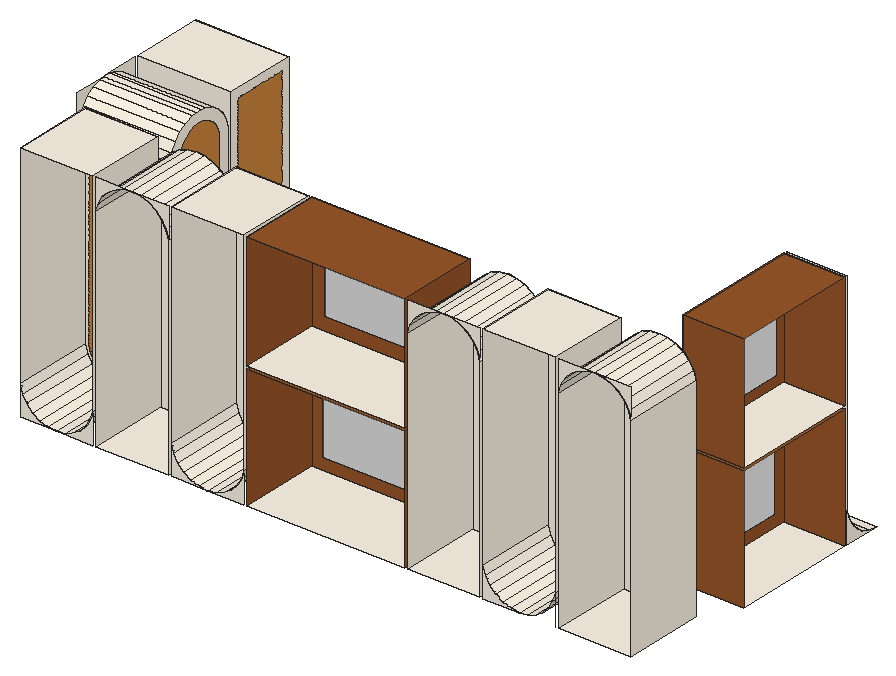
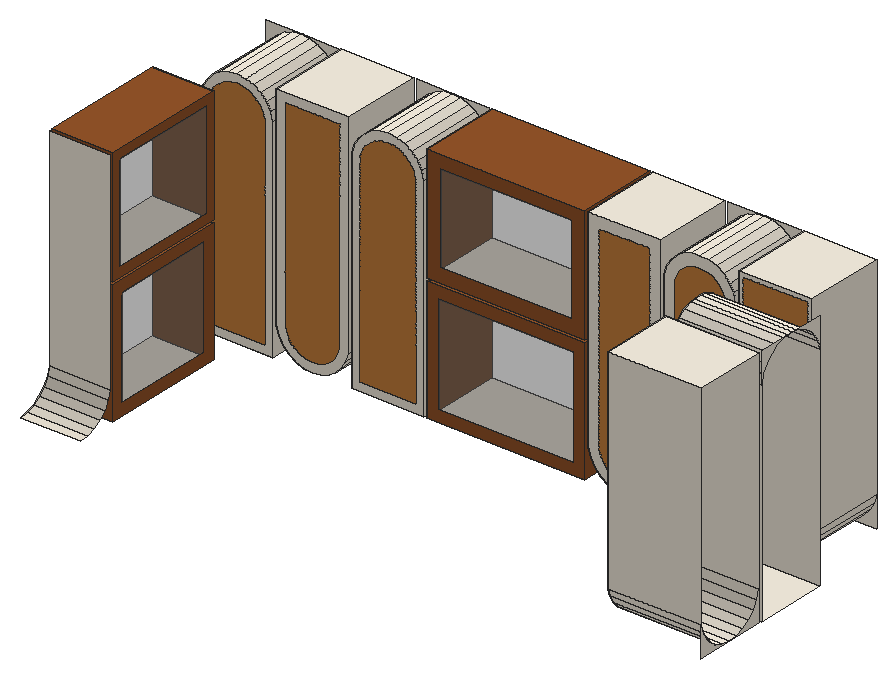
# SketchUp Ruby script. Lengths in inches.
U = 1.inch
M = Sketchup.active_model
def pt(a) = Geom::Point3d.new(a.map { |v| v * U })
def face(e, loops, mat)
  f = e.add_face(loops[0].map { |a| pt(a) })
  loops[1..].each { |l| e.add_face(l.map { |a| pt(a) }).erase! }
  f.material = f.back_material = mat if mat
  f
end
# faces: each face lists its corners as indices into pts; further lists are holes
def faces(e, pts, list, mat = nil) = list.each { |f| face(e, (f[0].is_a?(Array) ? f : [f]).map { |l| l.map { |i| pts[i] } }, mat) }
# xy, xz, yz: faces in a plane at the given z, y or x. An outline is a flat list of corners, or four numbers for a rectangle; further outlines are holes
def ring(l) = l.size == 4 ? [[l[0], l[1]], [l[2], l[1]], [l[2], l[3]], [l[0], l[3]]] : l.each_slice(2).to_a
def flat(e, list, mat, &to3) = list.each { |f| face(e, (f[0].is_a?(Array) ? f : [f]).map { |l| ring(l).map { |u, v| to3.(u, v) } }, mat) }
def xy(e, z, list, mat = nil) = flat(e, list, mat) { |x, y| [x, y, z] }
def xz(e, y, list, mat = nil) = flat(e, list, mat) { |x, z| [x, y, z] }
def yz(e, x, list, mat = nil) = flat(e, list, mat) { |y, z| [x, y, z] }
def lines(e, pts, list) = list.each { |a, b| e.add_line(pt(pts[a]), pt(pts[b])) }
# prism: a flat outline (further loops are holes) pulled along v
def prism(e, loops, v, mat = nil)
  f = face(e, loops, mat); d = Geom::Vector3d.new(v.map { |x| x * U })
  f.pushpull(f.normal.samedirection?(d) ? d.length : -d.length)
end
def box(e, o, s, mat = nil) = prism(e, [[o, [o[0] + s[0], o[1], o[2]], [o[0] + s[0], o[1] + s[1], o[2]], [o[0], o[1] + s[1], o[2]]]], [0, 0, s[2]], mat)
def at(x, y, z, deg = 0) = Geom::Transformation.translation(pt([x, y, z])) * Geom::Transformation.rotation(ORIGIN, Z_AXIS, deg.degrees)
def axes(o, x, y, z) = Geom::Transformation.new([*x, 0, *y, 0, *z, 0, *pt(o).to_a, 1])
def part(name) = M.definitions.add(name)
# library, detail: a bought-in or finely detailed component or shape, given as its bounding box
def library(name, o, s) = part(name).tap { |d| box(d.entities, o, s) }
def detail(e, o, s) = box(e.add_group.entities, o, s)
def put(e, d, t, mat = nil) = e.add_instance(d, t).tap { |i| i.material = mat if mat }
def group(e, t, mat = nil) = e.add_group.tap { |g| g.transformation = t; g.material = mat if mat }.entities
root = M.entities
M.materials.add("[0030_OldLace]").color = [253, 245, 230]
M.materials.add("[0040_Peru]").color = [205, 133, 63]
M.materials.add("[Translucent Glass Gray]").color = [128, 128, 128]
M.materials["[Translucent Glass Gray]"].alpha = 0.5
M.materials.add("[Wood Cherry Original]").color = [152, 86, 42]
xy(root,67.4375,[[9,29.46,24.375,41.46]],"[0030_OldLace]")
xy(root,67.6875,[[24.875,13.46,36.875,26.84],[49.875,13.46,76,26.84],[76.5,13.46,88.5,26.84],[101.5,13.46,113.5,26.84]],"[0030_OldLace]")
xy(root,67.8125,[[106.9375,32.34,117,53.28]],"[0030_OldLace]")
xy(root,87.9375,[[49.875,13.46,76,26.84]],"[Wood Cherry Original]")
xy(root,88.125,[[106.9375,32.34,117,53.28]],"[Wood Cherry Original]")
xy(root,88.4375,[[49.875,13.46,76,26.84]],"[0030_OldLace]")
xy(root,88.625,[[106.9375,32.34,117,53.28]],"[0030_OldLace]")
xy(root,107.5625,[[9,34.93,24.375,36],[9,41.96,24.375,53.96]],"[0030_OldLace]")
xy(root,107.625,[[12.375,13.46,24.375,26.84],[37.375,13.46,49.375,26.84]],"[0030_OldLace]")
xy(root,107.625,[[49.875,13.46,76,26.84]],"[Wood Cherry Original]")
xy(root,107.6875,[[89,13.46,101,26.84]],"[0030_OldLace]")
xy(root,107.6875,[[106.9375,32.34,117,53.28]],"[Wood Cherry Original]")
xz(root,13.46,[[12.375,67.6875,12.375,72.6875,12.79,71.34,13.5,70.12,14.47,69.1,15.65,68.33,16.97,67.85,18.375,67.6875],[18.375,67.6875,19.78,67.85,21.1,68.33,22.28,69.1,23.25,70.12,23.96,71.34,24.375,72.6875,24.375,67.6875],[37.375,67.6875,37.375,72.6875,37.79,71.34,38.5,70.12,39.47,69.1,40.65,68.33,41.97,67.85,43.375,67.6875],[43.375,67.6875,44.78,67.85,46.1,68.33,47.28,69.1,48.25,70.12,48.96,71.34,49.375,72.6875,49.375,67.6875],[89,67.6875,89,72.6875,89.41,71.34,90.125,70.12,91.09,69.1,92.27,68.33,93.6,67.85,95,67.6875],
  [24.875,102.625,24.875,107.625,30.875,107.625,29.47,107.46,28.15,106.98,26.97,106.21,26,105.19,25.29,103.97],[36.875,102.625,36.46,103.97,35.75,105.19,34.78,106.21,33.6,106.98,32.28,107.46,30.875,107.625,36.875,107.625],[76.5,102.625,76.5,107.625,82.5,107.625,81.1,107.46,79.77,106.98,78.59,106.21,77.625,105.19,76.91,103.97],[88.5,102.625,88.09,103.97,87.375,105.19,86.41,106.21,85.23,106.98,83.9,107.46,82.5,107.625,88.5,107.625],[101.5,102.625,101.5,107.625,107.5,107.625,106.1,107.46,104.77,106.98,103.59,106.21,102.625,105.19,101.91,103.97],
  [113.5,102.625,113.09,103.97,112.375,105.19,111.41,106.21,110.23,106.98,108.9,107.46,107.5,107.625,113.5,107.625]],"[0030_OldLace]")
xz(root,26.84,[[[18.375,67.6875,16.97,67.85,15.65,68.33,14.47,69.1,13.5,70.12,12.79,71.34,12.375,72.6875,12.375,107.625,24.375,107.625,24.375,72.6875,23.96,71.34,23.25,70.12,22.28,69.1,21.1,68.33,19.78,67.85],[18.375,68.33,19.625,68.48,20.8125,68.91,21.87,69.6,22.73,70.51,23.37,71.6,23.73,72.78,23.73,106.98,13.02,106.98,13.02,72.78,13.38,71.6,14.02,70.51,14.88,69.6,15.9375,68.91,17.125,68.48]],[[24.875,67.6875,24.875,102.625,25.29,103.97,26,105.19,26.97,106.21,28.15,106.98,29.47,107.46,30.875,107.625,32.28,107.46,33.6,106.98,34.78,106.21,35.75,105.19,36.46,103.97,36.875,102.625,36.875,67.6875],[26.64,69.46,35.11,69.46,35.11,102.36,34.83,103.26,34.33,104.12,33.64,104.84,32.8,105.39,31.87,105.73,30.875,105.84,29.88,105.73,28.95,105.39,28.11,104.84,27.42,104.12,26.92,103.26,26.64,102.36]],[[43.375,67.6875,41.97,67.85,40.65,68.33,39.47,69.1,38.5,70.12,37.79,71.34,37.375,72.6875,37.375,107.625,49.375,107.625,49.375,72.6875,48.96,71.34,48.25,70.12,47.28,69.1,46.1,68.33,44.78,67.85],[43.375,69.56,44.35,69.67,45.26,70,46.08,70.54,46.76,71.25,47.25,72.09,47.52,72.97,47.52,105.77,39.23,105.77,39.23,72.97,39.5,72.09,39.99,71.25,40.67,70.54,41.49,70,42.4,69.67]],[[76.5,67.6875,76.5,102.625,76.91,103.97,77.625,105.19,78.59,106.21,79.77,106.98,81.1,107.46,82.5,107.625,83.9,107.46,85.23,106.98,86.41,106.21,87.375,105.19,88.09,103.97,88.5,102.625,88.5,67.6875],[77.875,69.0625,87.125,69.0625,87.125,102.42,86.82,103.42,86.27,104.36,85.52,105.15,84.61,105.74,83.58,106.12,82.5,106.24,81.42,106.12,80.39,105.74,79.48,105.15,78.73,104.36,78.18,103.42,77.875,102.42]],[[95,67.6875,93.6,67.85,92.27,68.33,91.09,69.1,90.125,70.12,89.41,71.34,89,72.6875,89,107.6875,101,107.6875,101,72.6875,100.59,71.34,99.875,70.12,98.91,69.1,97.73,68.33,96.4,67.85],[95,69.14,96.07,69.26,97.08,69.625,97.98,70.21,98.72,70.99,99.26,71.92,99.5625,72.9,99.5625,106.25,90.4375,106.25,90.4375,72.9,90.74,71.92,91.28,70.99,92.02,70.21,92.92,69.625,93.93,69.26]],
  [[101.5,67.6875,101.5,102.625,101.91,103.97,102.625,105.19,103.59,106.21,104.77,106.98,106.1,107.46,107.5,107.625,108.9,107.46,110.23,106.98,111.41,106.21,112.375,105.19,113.09,103.97,113.5,102.625,113.5,67.6875],[102.875,69.0625,112.125,69.0625,112.125,102.42,111.82,103.42,111.27,104.36,110.52,105.15,109.61,105.75,108.58,106.12,107.5,106.24,106.42,106.12,105.39,105.75,104.48,105.15,103.73,104.36,103.18,103.42,102.875,102.42]]],"[0030_OldLace]")
xz(root,26.84,[[18.375,68.33,17.125,68.48,15.9375,68.91,14.88,69.6,14.02,70.51,13.38,71.6,13.02,72.78,13.02,106.98,23.73,106.98,23.73,72.78,23.37,71.6,22.73,70.51,21.87,69.6,20.8125,68.91,19.625,68.48],[77.875,69.0625,77.875,102.42,78.18,103.42,78.73,104.36,79.48,105.15,80.39,105.74,81.42,106.12,82.5,106.24,83.58,106.12,84.61,105.74,85.52,105.15,86.27,104.36,86.82,103.42,87.125,102.42,87.125,69.0625],[102.875,69.0625,102.875,102.42,103.18,103.42,103.73,104.36,104.48,105.15,105.39,105.75,106.42,106.12,107.5,106.24,108.58,106.12,109.61,105.75,110.52,105.15,111.27,104.36,111.82,103.42,112.125,102.42,112.125,69.0625],[95,69.14,93.93,69.26,92.92,69.625,92.02,70.21,91.28,70.99,90.74,71.92,90.4375,72.9,90.4375,106.25,99.5625,106.25,99.5625,72.9,99.26,71.92,98.72,70.99,97.98,70.21,97.08,69.625,96.07,69.26],[26.64,69.46,26.64,102.36,26.92,103.26,27.42,104.12,28.11,104.84,28.95,105.39,29.88,105.73,30.875,105.84,31.87,105.73,32.8,105.39,33.64,104.84,34.33,104.12,34.83,103.26,35.11,102.36,35.11,69.46],
  [43.375,69.56,42.4,69.67,41.49,70,40.67,70.54,39.99,71.25,39.5,72.09,39.23,72.97,39.23,105.77,47.52,105.77,47.52,72.97,47.25,72.09,46.76,71.25,46.08,70.54,45.26,70,44.35,69.67]],"[0040_Peru]")
xz(root,26.84,[[51.76,69.57,74.11,86.05],[52.125,90.6875,73.75,105.375]],"[Translucent Glass Gray]")
xz(root,26.84,[[[49.875,67.6875,76,87.9375],[51.76,69.57,74.11,86.05]],[[49.875,88.4375,76,107.625],[52.125,90.6875,73.75,105.375]]],"[Wood Cherry Original]")
xz(root,29.46,[[9,67.4375,24.375,102.5625]],"[0030_OldLace]")
xz(root,32.34,[[106.9375,67.8125,117,88.125],[106.9375,88.625,117,107.6875]],"[Wood Cherry Original]")
xz(root,41.46,[[9,67.4375,24.375,102.5625]],"[0030_OldLace]")
xz(root,41.96,[[9,72.4375,24.375,107.5625]],"[0030_OldLace]")
xz(root,53.28,[[106.9375,67.8125,117,88.125],[106.9375,88.625,117,107.6875]],"[Wood Cherry Original]")
xz(root,53.78,[[106.9375,72.8125,117,107.6875]],"[0030_OldLace]")
xz(root,53.96,[[9,72.4375,24.375,107.5625]],"[0030_OldLace]")
yz(root,9,[[41.96,67.4375,47.96,67.4375,46.56,67.6,45.24,68.08,44.06,68.85,43.09,69.87,42.38,71.09,41.96,72.4375],[47.96,67.4375,53.96,67.4375,53.96,72.4375,53.55,71.09,52.84,69.87,51.87,68.85,50.69,68.08,49.36,67.6],[29.46,102.5625,29.87,103.92,30.57,105.16,31.54,106.19,32.72,106.97,34.06,107.46,34.93,107.5625,29.46,107.5625],[41.46,102.5625,41.46,107.5625,36,107.5625,36.875,107.46,38.21,106.97,39.39,106.19,40.36,105.16,41.06,103.92],[34.93,107.5625,36,107.5625,35.46,107.625]],"[0030_OldLace]")
yz(root,12.375,[[13.46,72.6875,26.84,107.625]],"[0030_OldLace]")
yz(root,24.375,[[[29.46,67.4375,41.46,67.4375,41.46,102.5625,41.06,103.92,40.36,105.16,39.39,106.19,38.21,106.97,36.875,107.46,36,107.5625,34.93,107.5625,34.06,107.46,32.72,106.97,31.54,106.19,30.57,105.16,29.87,103.92,29.46,102.5625],[31.14,69.11,31.14,102.32,31.41,103.26,31.92,104.16,32.625,104.9,33.48,105.47,34.45,105.82,35.03,105.89,35.9,105.89,36.48,105.82,37.45,105.47,38.31,104.9,39.01,104.16,39.52,103.26,39.79,102.32,39.79,69.11]],[[47.96,67.4375,49.36,67.6,50.69,68.08,51.87,68.85,52.84,69.87,53.55,71.09,53.96,72.4375,53.96,107.5625,41.96,107.5625,41.96,72.4375,42.38,71.09,43.09,69.87,44.06,68.85,45.24,68.08,46.56,67.6],[47.96,68.93,46.91,69.05,45.91,69.42,45.02,70,44.28,70.77,43.75,71.6875,43.45,72.66,43.45,106.08,52.48,106.08,52.48,72.66,52.18,71.6875,51.65,70.77,50.91,70,50.02,69.42,49.02,69.05]],[13.46,72.6875,26.84,107.625]],"[0030_OldLace]")
yz(root,24.375,[[47.96,68.93,49.02,69.05,50.02,69.42,50.91,70,51.65,70.77,52.18,71.6875,52.48,72.66,52.48,106.08,43.45,106.08,43.45,72.66,43.75,71.6875,44.28,70.77,45.02,70,45.91,69.42,46.91,69.05],[31.14,69.11,39.79,69.11,39.79,102.32,39.52,103.26,39.01,104.16,38.31,104.9,37.45,105.47,36.48,105.82,35.9,105.89,35.03,105.89,34.45,105.82,33.48,105.47,32.625,104.9,31.92,104.16,31.41,103.26,31.14,102.32]],"[0040_Peru]")
yz(root,24.875,[[13.46,67.6875,26.84,102.625]],"[0030_OldLace]")
yz(root,36.875,[[13.46,67.6875,26.84,102.625]],"[0030_OldLace]")
yz(root,37.375,[[13.46,72.6875,26.84,107.625]],"[0030_OldLace]")
yz(root,49.375,[[13.46,72.6875,26.84,107.625]],"[0030_OldLace]")
yz(root,49.875,[[13.46,67.6875,26.84,87.9375],[13.46,88.4375,26.84,107.625]],"[Wood Cherry Original]")
yz(root,76,[[13.46,67.6875,26.84,87.9375],[13.46,88.4375,26.84,107.625]],"[Wood Cherry Original]")
yz(root,76.5,[[13.46,67.6875,26.84,102.625]],"[0030_OldLace]")
yz(root,88.5,[[13.46,67.6875,26.84,102.625]],"[0030_OldLace]")
yz(root,89,[[13.46,72.6875,26.84,107.6875]],"[0030_OldLace]")
yz(root,101,[[13.46,72.6875,26.84,107.6875]],"[0030_OldLace]")
yz(root,101.5,[[13.46,67.6875,26.84,102.625]],"[0030_OldLace]")
yz(root,106.9375,[[34.32,69.79,51.3,86.14],[33.83,90.12,51.79,106.2]],"[Translucent Glass Gray]")
yz(root,106.9375,[[[32.34,67.8125,53.28,88.125],[34.32,69.79,51.3,86.14]],[[32.34,88.625,53.28,107.6875],[33.83,90.12,51.79,106.2]]],"[Wood Cherry Original]")
yz(root,113.5,[[13.46,67.6875,26.84,102.625]],"[0030_OldLace]")
yz(root,117,[[53.78,67.8125,53.78,72.8125,54.19,71.46,54.9,70.25,55.87,69.23,57.05,68.46,58.38,67.98,59.78,67.8125]],"[0030_OldLace]")
p = [[9,46.56,67.6],[9,47.96,67.4375],[24.375,47.96,67.4375],[24.375,46.56,67.6],[9,49.36,67.6],[24.375,49.36,67.6],
  [9,45.24,68.08],[24.375,45.24,68.08],[9,50.69,68.08],[24.375,50.69,68.08],[18.375,13.46,67.6875],[16.97,13.46,67.85],
  [16.97,26.84,67.85],[18.375,26.84,67.6875],[19.78,13.46,67.85],[19.78,26.84,67.85],[43.375,13.46,67.6875],[41.97,13.46,67.85],
  [41.97,26.84,67.85],[43.375,26.84,67.6875],[44.78,13.46,67.85],[44.78,26.84,67.85],[95,13.46,67.6875],[93.6,13.46,67.85],
  [93.6,26.84,67.85],[95,26.84,67.6875],[96.4,13.46,67.85],[96.4,26.84,67.85],[117,59.78,67.8125],[117,58.38,67.98],
  [106.9375,58.38,67.98],[106.9375,59.78,67.8125],[15.65,13.46,68.33],[15.65,26.84,68.33],[21.1,13.46,68.33],[21.1,26.84,68.33],
  [40.65,13.46,68.33],[40.65,26.84,68.33],[46.1,13.46,68.33],[46.1,26.84,68.33],[92.27,13.46,68.33],[92.27,26.84,68.33],
  [97.73,13.46,68.33],[97.73,26.84,68.33],[117,57.05,68.46],[106.9375,57.05,68.46],[9,44.06,68.85],[24.375,44.06,68.85],
  [9,51.87,68.85],[24.375,51.87,68.85],[14.47,13.46,69.1],[14.47,26.84,69.1],[22.28,13.46,69.1],[22.28,26.84,69.1],
  [39.47,13.46,69.1],[39.47,26.84,69.1],[47.28,13.46,69.1],[47.28,26.84,69.1],[91.09,13.46,69.1],[91.09,26.84,69.1],
  [98.91,13.46,69.1],[98.91,26.84,69.1],[117,55.87,69.23],[106.9375,55.87,69.23],[9,43.09,69.87],[24.375,43.09,69.87],
  [9,52.84,69.87],[24.375,52.84,69.87],[13.5,13.46,70.12],[13.5,26.84,70.12],[23.25,13.46,70.12],[23.25,26.84,70.12],
  [38.5,13.46,70.12],[38.5,26.84,70.12],[48.25,13.46,70.12],[48.25,26.84,70.12],[90.125,13.46,70.12],[90.125,26.84,70.12],
  [99.875,13.46,70.12],[99.875,26.84,70.12],[117,54.9,70.25],[106.9375,54.9,70.25],[9,42.38,71.09],[24.375,42.38,71.09],
  [9,53.55,71.09],[24.375,53.55,71.09],[12.79,13.46,71.34],[12.79,26.84,71.34],[23.96,13.46,71.34],[23.96,26.84,71.34],
  [37.79,13.46,71.34],[37.79,26.84,71.34],[48.96,13.46,71.34],[48.96,26.84,71.34],[89.41,13.46,71.34],[89.41,26.84,71.34],
  [100.59,13.46,71.34],[100.59,26.84,71.34],[117,54.19,71.46],[106.9375,54.19,71.46],[9,41.96,72.4375],[24.375,41.96,72.4375],
  [9,53.96,72.4375],[24.375,53.96,72.4375],[12.375,13.46,72.6875],[12.375,26.84,72.6875],[24.375,13.46,72.6875],[24.375,26.84,72.6875],
  [37.375,13.46,72.6875],[37.375,26.84,72.6875],[49.375,13.46,72.6875],[49.375,26.84,72.6875],[89,13.46,72.6875],[89,26.84,72.6875],
  [101,13.46,72.6875],[101,26.84,72.6875],[117,53.78,72.8125],[106.9375,53.78,72.8125],[24.875,13.46,102.625],[25.29,13.46,103.97],
  [25.29,26.84,103.97],[24.875,26.84,102.625],[36.46,13.46,103.97],[36.875,13.46,102.625],[36.875,26.84,102.625],[36.46,26.84,103.97],
  [76.5,13.46,102.625],[76.91,13.46,103.97],[76.91,26.84,103.97],[76.5,26.84,102.625],[88.09,13.46,103.97],[88.5,13.46,102.625],
  [88.5,26.84,102.625],[88.09,26.84,103.97],[101.5,13.46,102.625],[101.91,13.46,103.97],[101.91,26.84,103.97],[101.5,26.84,102.625],
  [113.09,13.46,103.97],[113.5,13.46,102.625],[113.5,26.84,102.625],[113.09,26.84,103.97],[9,29.87,103.92],[9,29.46,102.5625],
  [24.375,29.46,102.5625],[24.375,29.87,103.92],[9,41.46,102.5625],[9,41.06,103.92],[24.375,41.06,103.92],[24.375,41.46,102.5625],
  [9,30.57,105.16],[24.375,30.57,105.16],[9,40.36,105.16],[24.375,40.36,105.16],[26,13.46,105.19],[26,26.84,105.19],
  [35.75,13.46,105.19],[35.75,26.84,105.19],[77.625,13.46,105.19],[77.625,26.84,105.19],[87.375,13.46,105.19],[87.375,26.84,105.19],
  [102.625,13.46,105.19],[102.625,26.84,105.19],[112.375,13.46,105.19],[112.375,26.84,105.19],[26.97,13.46,106.21],[26.97,26.84,106.21],
  [34.78,13.46,106.21],[34.78,26.84,106.21],[78.59,13.46,106.21],[78.59,26.84,106.21],[86.41,13.46,106.21],[86.41,26.84,106.21],
  [103.59,13.46,106.21],[103.59,26.84,106.21],[111.41,13.46,106.21],[111.41,26.84,106.21],[9,31.54,106.19],[24.375,31.54,106.19],
  [9,39.39,106.19],[24.375,39.39,106.19],[28.15,13.46,106.98],[28.15,26.84,106.98],[33.6,13.46,106.98],[33.6,26.84,106.98],
  [79.77,13.46,106.98],[79.77,26.84,106.98],[85.23,13.46,106.98],[85.23,26.84,106.98],[104.77,13.46,106.98],[104.77,26.84,106.98],
  [110.23,13.46,106.98],[110.23,26.84,106.98],[9,32.72,106.97],[24.375,32.72,106.97],[9,38.21,106.97],[24.375,38.21,106.97],
  [29.47,13.46,107.46],[29.47,26.84,107.46],[32.28,13.46,107.46],[32.28,26.84,107.46],[81.1,13.46,107.46],[81.1,26.84,107.46],
  [83.9,13.46,107.46],[83.9,26.84,107.46],[106.1,13.46,107.46],[106.1,26.84,107.46],[108.9,13.46,107.46],[108.9,26.84,107.46],
  [9,34.06,107.46],[24.375,34.06,107.46],[9,36.875,107.46],[24.375,36.875,107.46],[30.875,13.46,107.625],[30.875,26.84,107.625],
  [82.5,13.46,107.625],[82.5,26.84,107.625],[107.5,13.46,107.625],[107.5,26.84,107.625],[9,34.93,107.5625],[24.375,34.93,107.5625],
  [9,36,107.5625],[24.375,36,107.5625],[101,13.46,67.6875]]
faces(root,p,[[0,1,2,3],[1,4,5,2],[6,0,3,7],[4,8,9,5],[10,11,12,13],[14,10,13,15],[16,17,18,19],[20,16,19,21],
  [22,23,24,25],[26,22,25,27],[28,29,30,31],[11,32,33,12],[34,14,15,35],[17,36,37,18],[38,20,21,39],[23,40,41,24],
  [42,26,27,43],[29,44,45,30],[46,6,7,47],[8,48,49,9],[32,50,51,33],[52,34,35,53],[36,54,55,37],[56,38,39,57],
  [40,58,59,41],[60,42,43,61],[44,62,63,45],[64,46,47,65],[48,66,67,49],[50,68,69,51],[70,52,53,71],[54,72,73,55],
  [74,56,57,75],[58,76,77,59],[78,60,61,79],[62,80,81,63],[82,64,65,83],[66,84,85,67],[68,86,87,69],[88,70,71,89],
  [72,90,91,73],[92,74,75,93],[76,94,95,77],[96,78,79,97],[80,98,99,81],[100,82,83,101],[84,102,103,85],[86,104,105,87],
  [106,88,89,107],[90,108,109,91],[110,92,93,111],[94,112,113,95],[114,96,97,115],[98,116,117,99],[118,119,120,121],[122,123,124,125],
  [126,127,128,129],[130,131,132,133],[134,135,136,137],[138,139,140,141],[142,143,144,145],[146,147,148,149],[150,142,145,151],[147,152,153,148],
  [119,154,155,120],[156,122,125,157],[127,158,159,128],[160,130,133,161],[135,162,163,136],[164,138,141,165],[154,166,167,155],[168,156,157,169],
  [158,170,171,159],[172,160,161,173],[162,174,175,163],[176,164,165,177],[178,150,151,179],[152,180,181,153],[166,182,183,167],[184,168,169,185],
  [170,186,187,171],[188,172,173,189],[174,190,191,175],[192,176,177,193],[194,178,179,195],[180,196,197,181],[182,198,199,183],[200,184,185,201],
  [186,202,203,187],[204,188,189,205],[190,206,207,191],[208,192,193,209],[210,194,195,211],[196,212,213,197],[198,214,215,199],[214,200,201,215],
  [202,216,217,203],[216,204,205,217],[206,218,219,207],[218,208,209,219],[220,210,211,221],[212,222,223,213]],"[0030_OldLace]")
lines(root,p,[[114,224]])
